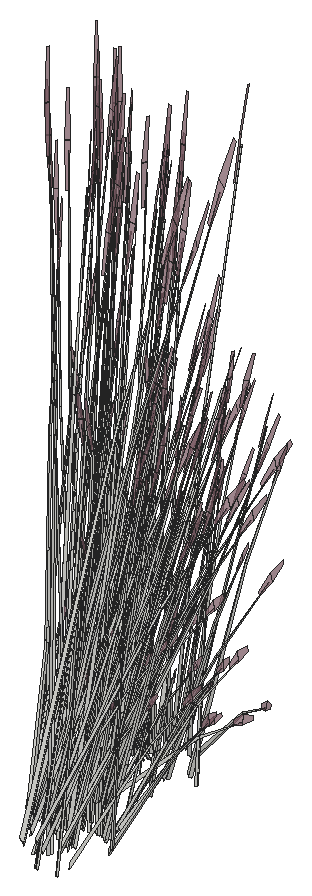
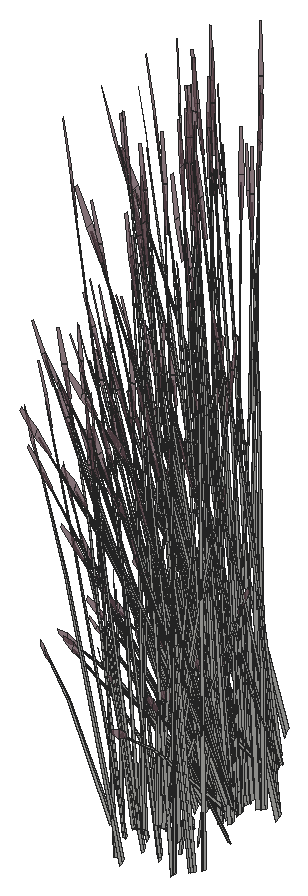
# SketchUp Ruby script. Lengths in inches.
U = 1.inch
M = Sketchup.active_model
def pt(a) = Geom::Point3d.new(a.map { |v| v * U })
def face(e, loops, mat)
  f = e.add_face(loops[0].map { |a| pt(a) })
  loops[1..].each { |l| e.add_face(l.map { |a| pt(a) }).erase! }
  f.material = f.back_material = mat if mat
  f
end
# faces: each face lists its corners as indices into pts; further lists are holes
def faces(e, pts, list, mat = nil) = list.each { |f| face(e, (f[0].is_a?(Array) ? f : [f]).map { |l| l.map { |i| pts[i] } }, mat) }
# xy, xz, yz: faces in a plane at the given z, y or x. An outline is a flat list of corners, or four numbers for a rectangle; further outlines are holes
def ring(l) = l.size == 4 ? [[l[0], l[1]], [l[2], l[1]], [l[2], l[3]], [l[0], l[3]]] : l.each_slice(2).to_a
def flat(e, list, mat, &to3) = list.each { |f| face(e, (f[0].is_a?(Array) ? f : [f]).map { |l| ring(l).map { |u, v| to3.(u, v) } }, mat) }
def xy(e, z, list, mat = nil) = flat(e, list, mat) { |x, y| [x, y, z] }
def xz(e, y, list, mat = nil) = flat(e, list, mat) { |x, z| [x, y, z] }
def yz(e, x, list, mat = nil) = flat(e, list, mat) { |y, z| [x, y, z] }
def lines(e, pts, list) = list.each { |a, b| e.add_line(pt(pts[a]), pt(pts[b])) }
# prism: a flat outline (further loops are holes) pulled along v
def prism(e, loops, v, mat = nil)
  f = face(e, loops, mat); d = Geom::Vector3d.new(v.map { |x| x * U })
  f.pushpull(f.normal.samedirection?(d) ? d.length : -d.length)
end
def box(e, o, s, mat = nil) = prism(e, [[o, [o[0] + s[0], o[1], o[2]], [o[0] + s[0], o[1] + s[1], o[2]], [o[0], o[1] + s[1], o[2]]]], [0, 0, s[2]], mat)
def at(x, y, z, deg = 0) = Geom::Transformation.translation(pt([x, y, z])) * Geom::Transformation.rotation(ORIGIN, Z_AXIS, deg.degrees)
def axes(o, x, y, z) = Geom::Transformation.new([*x, 0, *y, 0, *z, 0, *pt(o).to_a, 1])
def part(name) = M.definitions.add(name)
# library, detail: a bought-in or finely detailed component or shape, given as its bounding box
def library(name, o, s) = part(name).tap { |d| box(d.entities, o, s) }
def detail(e, o, s) = box(e.add_group.entities, o, s)
def put(e, d, t, mat = nil) = e.add_instance(d, t).tap { |i| i.material = mat if mat }
def group(e, t, mat = nil) = e.add_group.tap { |g| g.transformation = t; g.material = mat if mat }.entities
root = M.entities
M.materials.add("LightPink_Translucent").color = [144, 107, 117]
M.materials["LightPink_Translucent"].alpha = 0.75
c1 = part("blade")
p = [[2.15,0.21,22],[0,0.17,0],[0.09,0.45,0],[2.18,0.31,22],[2.29,0.31,22],[0.38,0.45,0],
  [2.48,0.24,33],[2.49,0.24,33],[2.48,0.22,33]]
faces(c1.entities,p,[[0,1,2,3],[4,5,2,3],[6,3,4,7],[8,0,3,6]])
c2 = part("seeds")
p = [[0.3,-0.1,1.38],[-0.01,-0.03,1.59],[-0.01,-0.03,0.03],[0.14,-0.07,-0.07],[0.29,-0.03,3],[0.15,0.01,3.11]]
faces(c2.entities,p,[[0,1,2,3],[1,0,4,5]],"LightPink_Translucent")
c3 = part("blade with seeds")
put(c3.entities,c1,at(0,0,0))
put(c3.entities,c2,axes([2.4,0.25,30.99],[1.5799,-0.05474,1.17369],[-0.12525,1.92788,0.29478],[-0.07173,-0.02425,1.56792]))
put(root,c3,axes([688.9,323.21,391.83],[-0.21227,-0.49226,0],[0.60616,-0.17239,0],[0,0,1.28128]))
put(root,c3,axes([688.125,324.25,391.24],[0.10529,-0.03107,1.46364],[0.63335,0.17101,-0.2236],[0.01852,0.19274,0.24931]))
put(root,c3,axes([688.98,318.93,394.2],[-0.64106,-0.14927,0.44225],[0.21921,-0.49074,0.36465],[0.03852,0.19299,0.91512]))
put(root,c3,axes([688.26,324.42,393.76],[-0.19614,0.43908,-0.29394],[-0.57222,-0.12807,0.37948],[0.05247,0.17678,0.72609]))
put(root,c3,axes([688.81,318.97,393.93],[-0.47939,0.19405,0.05337],[-0.23464,-0.35385,0.42015],[0.0463,0.15598,0.64067]))
put(root,c3,axes([686.58,328.93,391.97],[-0.40676,-0.57214,0],[0.68052,-0.31907,-0.42834],[0.15499,-0.07267,1.3588]))
put(root,c3,axes([689.75,322.24,391.83],[-0.31565,0.51449,-0.37133],[-0.65588,-0.24761,0.17871],[0,0.1186,1.19224]))
put(root,c3,axes([688.28,327.55,392.3],[0.08346,0.33295,0.95334],[-0.46298,-0.1844,0.70045],[0.04982,-0.17048,0.20998]))
put(root,c3,axes([690.55,318.33,391.93],[0.81449,0.18558,0.25528],[-0.20377,0.66335,-0.30288],[-0.13481,0.08302,1.36855]))
put(root,c3,axes([687.86,325.2,393.91],[0.08247,0.09194,1.45204],[0.66552,0.03612,-0.22964],[0.06692,0.20277,0.11645]))
put(root,c3,axes([691,321.93,392.05],[-0.51116,-0.4159,0.14643],[0.51512,-0.4034,0.29122],[-0.05645,0.08494,1.33138]))
put(root,c3,axes([689.23,321.6875,391.83],[0,-0.66065,0],[0.81352,0,0],[0,0,1.48949]))
put(root,c3,axes([689.64,321.95,391.9],[0,0.66033,-0.04679],[-0.81352,0,0],[0,0.02075,1.48875]))
put(root,c3,axes([688.24,321.42,392.26],[-0.70648,0.03525,0.37133],[-0.06389,-0.58508,-0.17871],[0.12647,-0.0593,1.19224]))
put(root,c3,axes([688.91,318.86,391.24],[0.10529,-0.03107,1.46364],[0.63335,0.17101,-0.2236],[0.01852,0.19274,0.24931]))
put(root,c3,axes([688.2,323.96,394.19],[0.19614,-0.43908,0.29394],[0.57222,0.12807,-0.37948],[0.05247,0.17678,0.72609]))
put(root,c3,axes([689.05,319.04,393.76],[-0.19614,0.43908,-0.29394],[-0.57222,-0.12807,0.37948],[0.05247,0.17678,0.72609]))
put(root,c3,axes([690.27,328.09,393.91],[-0.06607,0.04361,1.47228],[-0.64734,-0.14714,-0.13912],[-0.02343,-0.19032,0.26054]))
put(root,c3,axes([689.76,329.35,394.18],[-0.71502,-0.02829,-0.10093],[0.01954,-0.53563,-0.56021],[0.04967,-0.20629,0.85122]))
put(root,c3,axes([687.91,320.42,392.05],[-0.18794,0.56744,0.14643],[-0.68774,-0.16058,0.29122],[0.1188,-0.00276,1.33138]))
put(root,c3,axes([689.25,323.23,391.9],[0.28286,0.65594,-0.0499],[-0.80821,0.22985,0],[0.00988,0.02291,1.42904]))
put(root,c3,axes([689.48,329.43,394.19],[-0.4402,0.30062,0.29394],[-0.41671,-0.34326,-0.37948],[0.0634,-0.1744,0.72609]))
put(root,c3,axes([687.38,330.51,392.21],[-0.07581,-0.65151,-0.24149],[0.7896,-0.03939,-0.41502],[0.13904,-0.08678,1.32557]))
put(root,c3,axes([688.32,324.03,394.13],[0.31051,0.46426,-0.58968],[-0.63919,0.25873,0.07116],[0.07261,0.22432,0.83415]))
put(root,c3,axes([691.59,322.37,391.83],[-0.81312,-0.00457,-0.0413],[0,-0.63814,0.41452],[-0.02555,0.14527,1.31432]))
put(root,c3,axes([689.27,329.15,393.89],[-0.46573,-0.38364,-0.42412],[0.49199,-0.33598,-0.32852],[0.07086,-0.19492,0.81151]))
put(root,c3,axes([689.99,320.45,392.05],[-0.6991,0.15154,0.14643],[-0.17263,-0.56398,0.29122],[0.06235,0.08217,1.33138]))
put(root,c3,axes([688.64,319.8125,393.91],[0.08247,0.09194,1.45204],[0.66552,0.03612,-0.22964],[0.06692,0.20277,0.11645]))
put(root,c3,axes([688.97,325.53,394.6875],[0.44958,-0.32756,-0.05385],[0.41194,0.35875,-0.24415],[0.029,0.10165,0.8053]))
put(root,c3,axes([688.85,321.27,391.96],[-0.53943,0.51816,0.37976],[-0.64086,-0.4574,0.14902],[0.13005,-0.05171,1.31851]))
put(root,c3,axes([689.77,322.09,391.84],[0.45414,0.3688,0],[-0.45414,0.3688,0],[0,0,1.40491]))
put(root,c3,axes([687.27,329.07,391.68],[0.60696,0.14127,-0.25712],[-0.15283,0.49751,0.25712],[0.12236,-0.05737,1.15348]))
put(root,c3,axes([688.99,318.57,394.19],[0.19614,-0.43908,0.29394],[0.57222,0.12807,-0.37948],[0.05247,0.17678,0.72609]))
put(root,c3,axes([689.76,321.66,392.26],[0.31565,-0.51449,0.37133],[0.65588,0.24761,-0.17871],[0,0.1186,1.19224]))
put(root,c3,axes([689.49,323.44,391.83],[0.65588,0.25634,0],[-0.31565,0.53263,0],[0,0,1.45212]))
put(root,c3,axes([688.96,328.47,392.15],[-0.18493,0.11557,1.18691],[-0.55384,-0.20228,-0.25526],[0.10266,-0.25157,0.50747]))
put(root,c3,axes([688.56,324.12,393.89],[0.63954,0.14313,-0.42412],[-0.21921,0.49074,-0.32852],[0.05864,0.19758,0.81151]))
put(root,c3,axes([688.01,324.15,394.18],[0.63664,-0.26583,-0.10093],[0.31286,0.47181,-0.56021],[0.084,0.19882,0.85122]))
put(root,c3,axes([689.55,321.53,391.98],[-0.82229,-0.1203,0.40835],[0.16734,-0.67942,0.16024],[0.12017,0.06561,1.41775]))
put(root,c3,axes([687.13,328.84,391.67],[0.60889,-0.28548,-0.4121],[0.36394,0.51192,0],[0.13868,-0.06502,1.30728]))
put(root,c3,axes([691.42,322.46,391.68],[-0.45414,0.35624,-0.25712],[-0.45414,-0.35624,0.25712],[0,0.11474,1.15348]))
put(root,c3,axes([689.11,318.64,394.13],[0.31051,0.46426,-0.58968],[-0.63919,0.25873,0.07116],[0.07261,0.22432,0.83415]))
put(root,c3,axes([690.125,322.39,391.74],[0.23855,0.52277,-0.57446],[-0.68718,0.18827,-0.15077],[0.02637,0.17702,1.26801]))
put(root,c3,axes([689.79,321.83,391.83],[0.72788,0,0],[0,0.59111,0],[0,0,1.48078]))
put(root,c3,axes([689.09,321.18,392.26],[-0.39083,-0.47924,0.37133],[0.59199,-0.33747,-0.17871],[0.12647,0.0593,1.19224]))
put(root,c3,axes([689.41,329.32,394.13],[0.01693,-0.52814,-0.58968],[0.71285,0.03547,0.07116],[0.07523,-0.22375,0.83415]))
put(root,c3,axes([690.04,321.77,392.17],[0.60616,-0.16651,0.12018],[0.21227,0.47548,-0.34318],[0,0.10465,1.05198]))
put(root,c3,axes([689.76,320.14,394.6875],[0.44958,-0.32756,-0.05385],[0.41194,0.35875,-0.24415],[0.029,0.10165,0.8053]))
put(root,c3,axes([689.83,321.8125,392.21],[0.73268,0.27244,-0.24149],[-0.35279,0.57501,-0.41502],[0.02303,0.14118,1.32557]))
put(root,c3,axes([689.34,318.74,393.89],[0.63954,0.14313,-0.42412],[-0.21921,0.49074,-0.32852],[0.05864,0.19758,0.81151]))
put(root,c3,axes([688.79,318.76,394.18],[0.63664,-0.26583,-0.10093],[0.31286,0.47181,-0.56021],[0.084,0.19882,0.85122]))
put(root,c3,axes([691.42,321.94,392.06],[0,-0.57097,0.4121],[0.72788,0,0],[0,0.13004,1.30728]))
put(root,c3,axes([689.71,329.01,393.76],[0.4402,-0.30062,-0.29394],[0.41671,0.34326,0.37948],[0.0634,-0.1744,0.72609]))
put(root,c3,axes([691.73,322.47,391.67],[0,0.57097,-0.4121],[-0.72788,0,0],[0,0.13004,1.30728]))
put(root,c3,axes([690.91,317.01,391.74],[0.23855,0.52277,-0.57446],[-0.68718,0.18827,-0.15077],[0.02637,0.17702,1.26801]))
put(root,c3,axes([689.79,324.2,393.93],[-0.64708,0.13103,0.39842],[-0.1123,-0.514,0.32852],[0.15218,0.15149,0.82444]))
put(root,c3,axes([689.67,324.3,393.93],[-0.29569,0.36271,0.05337],[-0.42107,-0.21117,0.42015],[0.13613,0.11629,0.64067]))
put(root,c3,axes([689.875,329.16,393.93],[0.53464,0.0266,0.05337],[-0.01466,0.40172,0.42015],[0.05594,-0.15388,0.64067]))
put(root,c3,axes([688.92,323.11,393.22],[-0.14872,-0.18332,1.42242],[0.6872,-0.15433,0.11501],[0.15531,0.28779,0.60807]))
put(root,c3,axes([689.35,321.05,392.17],[0.12551,-0.50956,0.12018],[0.6132,0.08845,-0.34318],[0.1116,0.05232,1.05198]))
put(root,c3,axes([690.41,328.5,393.91],[-0.00628,-0.11364,1.45204],[-0.53042,-0.32843,-0.22964],[0.08201,-0.19909,0.11645]))
put(root,c3,axes([687.85,330.01,391.71],[0.43821,-0.42916,-0.51753],[0.54436,0.38915,-0.13583],[0.1756,-0.10706,1.14236]))
put(root,c3,axes([689.71,329.125,393.93],[0.46327,0.38957,0.39842],[-0.49199,0.33598,0.32852],[0.08546,-0.18277,0.82444]))
put(root,c3,axes([690.22,320.16,392.06],[-0.60889,-0.28548,0.4121],[0.36394,-0.51192,0],[0.13868,0.06502,1.30728]))
put(root,c3,axes([689.69,323.14,391.8125],[0.68303,-0.19373,-0.15934],[0.24001,0.55805,0.00007],[0.07539,-0.02141,1.44335]))
put(root,c3,axes([690.24,330.36,394.19],[-0.56631,0.0816,0.29394],[-0.14954,-0.46647,-0.37948],[0.16229,-0.12529,0.72609]))
put(root,c3,axes([689.57,323.89,394.19],[-0.10048,-0.4599,0.29394],[0.5744,-0.12144,-0.37948],[0.15428,0.13179,0.72609]))
put(root,c3,axes([692.52,317.09,391.67],[0,0.57097,-0.4121],[-0.72788,0,0],[0,0.13004,1.30728]))
put(root,c3,axes([690.57,318.82,393.93],[-0.64708,0.13103,0.39842],[-0.1123,-0.514,0.32852],[0.15218,0.15149,0.82444]))
put(root,c3,axes([690.45,318.92,393.93],[-0.29569,0.36271,0.05337],[-0.42107,-0.21117,0.42015],[0.13613,0.11629,0.64067]))
put(root,c3,axes([689.7,321.48,391.83],[0.39083,0.47924,-0.37133],[-0.59199,0.33747,0.17871],[0.12647,0.0593,1.19224]))
put(root,c3,axes([689.7,317.72,393.22],[-0.14872,-0.18332,1.42242],[0.6872,-0.15433,0.11501],[0.15531,0.28779,0.60807]))
put(root,c3,axes([688.61,329.06,393.22],[-0.12114,0.19625,1.42242],[-0.50818,-0.40613,0.11501],[0.22925,-0.25313,0.60807]))
put(root,c3,axes([689.96,321.24,393.71],[-0.56218,-0.29666,1.14775],[0.59361,-0.46189,0.49522],[0.18138,0.27836,1.10941]))
put(root,c3,axes([689.02,324.53,393.91],[0.00193,-0.06913,1.47228],[0.55753,-0.30498,-0.13912],[0.19366,0.10886,0.26054]))
put(root,c3,axes([690.81,323.66,392.3],[-0.36631,-0.16417,0.95334],[0.47299,-0.16681,0.70045],[0.12758,0.1413,0.20998]))
put(root,c3,axes([689.51,323.48,392.15],[0.01148,-0.18927,1.18691],[0.54864,-0.21141,-0.25526],[0.16937,0.22654,0.50747]))
put(root,c3,axes([690.53,330.4,394.18],[-0.60181,-0.31483,-0.10093],[0.34671,-0.45593,-0.56021],[0.17003,-0.15849,0.85122]))
put(root,c3,axes([690.77,320.42,391.68],[0.15283,0.49751,-0.25712],[-0.60696,0.14127,0.25712],[0.12236,0.05737,1.15348]))
put(root,c3,axes([691.92,322.04,391.97],[0.81352,0,0],[0,0.63814,-0.42834],[0,0.14534,1.3588]))
put(root,c3,axes([689.57,329.07,391.97],[0.40676,-0.57214,0],[0.68052,0.31907,-0.42834],[0.15499,0.07267,1.3588]))
put(root,c3,axes([690.26,328.82,391.24],[-0.09738,-0.04498,1.46364],[-0.25012,-0.50252,-0.2236],[0.16873,-0.13637,0.24931]))
put(root,c3,axes([690.36,318.5,394.19],[-0.10048,-0.4599,0.29394],[0.5744,-0.12144,-0.37948],[0.15428,0.13179,0.72609]))
put(root,c3,axes([689.29,321.21,392.21],[0.65687,-0.37907,-0.24149],[0.43681,0.53562,-0.41502],[0.16207,0.0544,1.32557]))
put(root,c3,axes([690.87,324.4,392.21],[-0.4172,-0.01791,0.872],[0.27552,-0.38032,0.48145],[0.16481,0.13512,0.68401]))
put(root,c3,axes([690.75,315.86,393.71],[-0.56218,-0.29666,1.14775],[0.59361,-0.46189,0.49522],[0.18138,0.27836,1.10941]))
put(root,c3,axes([690.24,330.03,393.89],[-0.16713,-0.52135,-0.42412],[0.63294,-0.0912,-0.32852],[0.18138,-0.14003,0.81151]))
put(root,c3,axes([689.8,319.14,393.91],[0.00193,-0.06913,1.47228],[0.55753,-0.30498,-0.13912],[0.19366,0.10886,0.26054]))
put(root,c3,axes([691.59,318.27,392.3],[-0.36631,-0.16417,0.95334],[0.47299,-0.16681,0.70045],[0.12758,0.1413,0.20998]))
put(root,c3,axes([690.29,318.1,392.15],[0.01148,-0.18927,1.18691],[0.54864,-0.21141,-0.25526],[0.16937,0.22654,0.50747]))
put(root,c3,axes([691.9375,330.85,391.875],[-0.40335,-0.3651,-0.05385],[0.44175,-0.33453,-0.24415],[0.12517,-0.02355,0.8053]))
put(root,c3,axes([689.52,324.125,394.18],[0.38768,-0.48872,-0.10093],[0.56143,0.28156,-0.56021],[0.19516,0.13808,0.85122]))
put(root,c3,axes([687.63,320.875,391.32],[-0.64037,0.22859,1.07011],[-0.20382,-0.65589,0.4158],[0.39323,0.01091,1.21713]))
put(root,c3,axes([691.01,328.99,392.3],[-0.2167,0.29065,0.95334],[-0.18626,-0.3905,0.70045],[0.17898,-0.09785,0.20998]))
put(root,c3,axes([690.75,330.29,393.93],[0.44663,0.24013,0.05337],[-0.26003,0.34195,0.42015],[0.14319,-0.11055,0.64067]))
put(root,c3,axes([689.98,323.88,393.89],[0.64198,-0.13573,-0.42412],[0.1123,0.514,-0.32852],[0.17243,0.1473,0.81151]))
put(root,c3,axes([691.65,319.02,392.21],[-0.4172,-0.01791,0.872],[0.27552,-0.38032,0.48145],[0.16481,0.13512,0.68401]))
put(root,c3,axes([690.57,319.86,391.97],[0.40676,-0.57214,0],[0.68052,0.31907,-0.42834],[0.15499,0.07267,1.3588]))
put(root,c3,axes([690.63,330.1875,393.93],[0.16135,0.52549,0.39842],[-0.63294,0.0912,0.32852],[0.18654,-0.12359,0.82444]))
put(root,c3,axes([690.72,323.27,394.19],[-0.37017,-0.35748,0.29394],[0.42268,-0.3384,-0.37948],[0.21476,0.05149,0.72609]))
put(root,c3,axes([690.94,320.21,391.67],[0.60889,0.28548,-0.4121],[-0.36394,0.51192,0],[0.13868,0.06502,1.30728]))
put(root,c3,axes([691.05,323.59,393.93],[-0.03276,0.43418,0.05337],[-0.49468,-0.0119,0.42015],[0.18949,0.04543,0.64067]))
put(root,c3,axes([690.91,324.27,391.24],[0.0474,-0.08243,1.46364],[0.59674,-0.24277,-0.2236],[0.18092,0.12565,0.24931]))
put(root,c3,axes([692.02,330.27,393.91],[-0.08498,-0.00434,1.47228],[-0.35287,-0.46464,-0.13912],[0.14171,-0.15278,0.26054]))
put(root,c3,axes([691.1,323.45,393.93],[-0.47971,0.37622,0.39842],[-0.41372,-0.39954,0.32852],[0.22506,0.0694,0.82444]))
put(root,c3,axes([690.7,330.09,393.76],[0.56631,-0.0816,-0.29394],[0.14954,0.46647,0.37948],[0.16229,-0.12529,0.72609]))
put(root,c3,axes([692.35,323.51,393.26],[-0.12452,-0.47997,-0.02898],[0.58854,-0.11034,-0.1314],[0.1229,0.03043,0.43341]))
put(root,c3,axes([690.31,318.74,394.18],[0.38768,-0.48872,-0.10093],[0.56143,0.28156,-0.56021],[0.19516,0.13808,0.85122]))
put(root,c3,axes([691.33,322.26,394.19],[-0.54068,-0.15928,0.29394],[0.1577,-0.46469,-0.37948],[0.21769,-0.04261,0.72609]))
put(root,c3,axes([690.25,330.24,394.13],[0.33983,-0.45051,-0.58968],[0.59551,0.32017,0.07116],[0.20291,-0.16322,0.83415]))
put(root,c3,axes([690.56,331.63,394.18],[-0.32734,-0.51701,-0.10093],[0.58097,-0.25407,-0.56021],[0.24483,-0.06821,0.85122]))
put(root,c3,axes([690.05,321.3,391.71],[0.67676,0.09361,-0.51753],[-0.14281,0.57742,-0.13583],[0.20196,0.06997,1.14236]))
put(root,c3,axes([692.9375,321.64,391.875],[-0.40335,-0.3651,-0.05385],[0.44175,-0.33453,-0.24415],[0.12517,-0.02355,0.8053]))
put(root,c3,axes([690.77,318.5,393.89],[0.64198,-0.13573,-0.42412],[0.1123,0.514,-0.32852],[0.17243,0.1473,0.81151]))
put(root,c3,axes([691.7,318.88,391.24],[0.0474,-0.08243,1.46364],[0.59674,-0.24277,-0.2236],[0.18092,0.12565,0.24931]))
put(root,c3,axes([689.91,322.54,393.22],[-0.24166,-0.09837,1.42242],[0.50011,-0.41269,0.11501],[0.3117,0.18617,0.60807]))
put(root,c3,axes([690.53,331.1875,393.89],[0.17625,-0.51936,-0.42412],[0.60429,0.17802,-0.32852],[0.2433,-0.04762,0.81151]))
put(root,c3,axes([690.75,329.83,392.15],[-0.23242,-0.01691,1.18691],[-0.23811,-0.45367,-0.25526],[0.28553,-0.12834,0.50747]))
put(root,c3,axes([691.82,322.41,393.93],[0.23895,0.38931,0.05337],[-0.43573,0.19055,0.42015],[0.19208,-0.0376,0.64067]))
put(root,c3,axes([691.24,323.45,393.76],[0.37017,0.35748,-0.29394],[-0.42268,0.3384,0.37948],[0.21476,0.05149,0.72609]))
put(root,c3,axes([690.82,323.49,394.18],[0.03484,-0.58066,-0.10093],[0.65957,0.01587,-0.56021],[0.25402,0.04034,0.85122]))
put(root,c3,axes([691.56,322.42,394.18],[-0.32734,-0.51701,-0.10093],[0.58097,-0.25407,-0.56021],[0.24483,-0.06821,0.85122]))
put(root,c3,axes([691.77,322.27,393.93],[-0.18381,0.5206,0.39842],[-0.60429,-0.17802,0.32852],[0.23764,-0.03129,0.82444]))
put(root,c3,axes([691.18,331.34,391.65],[-0.41902,0.06852,1.17514],[-0.0667,-0.54541,0.06726],[0.29348,-0.08255,0.6687]))
put(root,c3,axes([690.7,317.15,393.22],[-0.24166,-0.09837,1.42242],[0.50011,-0.41269,0.11501],[0.3117,0.18617,0.60807]))
put(root,c3,axes([691.39,323.15,393.91],[0.13956,-0.00966,1.45204],[0.38281,-0.44358,-0.22964],[0.24825,0.05855,0.11645]))
put(root,c3,axes([691.53,321.98,393.89],[0.17625,-0.51936,-0.42412],[0.60429,0.17802,-0.32852],[0.2433,-0.04762,0.81151]))
put(root,c3,axes([693.04,322.31,392.3],[-0.40197,0.09426,0.95334],[0.18921,-0.38956,0.70045],[0.21325,0.02666,0.20998]))
put(root,c3,axes([692.34,330.82,393.91],[0.09028,-0.08697,1.45204],[-0.11555,-0.53348,-0.22964],[0.22652,-0.10115,0.11645]))
put(root,c3,axes([691.9,322.21,393.76],[0.54068,0.15928,-0.29394],[-0.1577,0.46469,0.37948],[0.21769,-0.04261,0.72609]))
put(root,c3,axes([690.85,323.21,394.13],[0.65035,0.01375,-0.58968],[-0.04368,0.5789,0.07116],[0.27552,0.06109,0.83415]))
put(root,c3,axes([692.17,322.12,391.65],[-0.41902,0.06852,1.17514],[-0.0667,-0.54541,0.06726],[0.29348,-0.08255,0.6687]))
put(root,c3,axes([692.63,321.77,391.24],[-0.034,-0.08668,1.46364],[0.23582,-0.50706,-0.2236],[0.23788,-0.00729,0.24931]))
put(root,c3,axes([692.86,323.96,393.91],[-0.05883,-0.04999,1.47228],[0.12868,-0.53581,-0.13912],[0.23172,-0.03423,0.26054]))
put(root,c3,axes([690.42,321.64,393.22],[-0.26985,0.01293,1.42242],[0.17902,-0.56047,0.11501],[0.38456,0.03467,0.60807]))
put(root,c3,axes([691.41,322.16,394.13],[0.57168,-0.25217,-0.58968],[0.3186,0.51908,0.07116],[0.27622,-0.05897,0.83415]))
put(root,c3,axes([692.29,322.93,392.15],[-0.15668,-0.14043,1.18691],[0.20386,-0.46454,-0.25526],[0.31701,0.06293,0.50747]))
